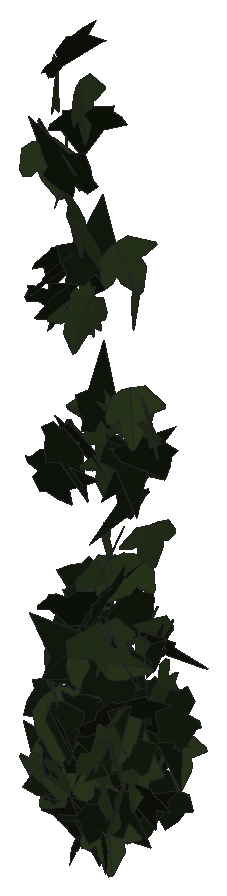
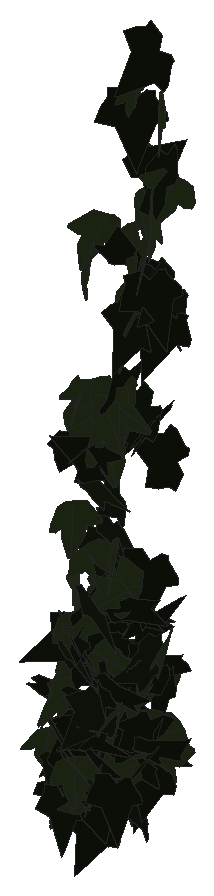
# SketchUp Ruby script. Lengths in inches.
U = 1.inch
M = Sketchup.active_model
def pt(a) = Geom::Point3d.new(a.map { |v| v * U })
def face(e, loops, mat)
  f = e.add_face(loops[0].map { |a| pt(a) })
  loops[1..].each { |l| e.add_face(l.map { |a| pt(a) }).erase! }
  f.material = f.back_material = mat if mat
  f
end
# faces: each face lists its corners as indices into pts; further lists are holes
def faces(e, pts, list, mat = nil) = list.each { |f| face(e, (f[0].is_a?(Array) ? f : [f]).map { |l| l.map { |i| pts[i] } }, mat) }
# xy, xz, yz: faces in a plane at the given z, y or x. An outline is a flat list of corners, or four numbers for a rectangle; further outlines are holes
def ring(l) = l.size == 4 ? [[l[0], l[1]], [l[2], l[1]], [l[2], l[3]], [l[0], l[3]]] : l.each_slice(2).to_a
def flat(e, list, mat, &to3) = list.each { |f| face(e, (f[0].is_a?(Array) ? f : [f]).map { |l| ring(l).map { |u, v| to3.(u, v) } }, mat) }
def xy(e, z, list, mat = nil) = flat(e, list, mat) { |x, y| [x, y, z] }
def xz(e, y, list, mat = nil) = flat(e, list, mat) { |x, z| [x, y, z] }
def yz(e, x, list, mat = nil) = flat(e, list, mat) { |y, z| [x, y, z] }
def lines(e, pts, list) = list.each { |a, b| e.add_line(pt(pts[a]), pt(pts[b])) }
# prism: a flat outline (further loops are holes) pulled along v
def prism(e, loops, v, mat = nil)
  f = face(e, loops, mat); d = Geom::Vector3d.new(v.map { |x| x * U })
  f.pushpull(f.normal.samedirection?(d) ? d.length : -d.length)
end
def box(e, o, s, mat = nil) = prism(e, [[o, [o[0] + s[0], o[1], o[2]], [o[0] + s[0], o[1] + s[1], o[2]], [o[0], o[1] + s[1], o[2]]]], [0, 0, s[2]], mat)
def at(x, y, z, deg = 0) = Geom::Transformation.translation(pt([x, y, z])) * Geom::Transformation.rotation(ORIGIN, Z_AXIS, deg.degrees)
def axes(o, x, y, z) = Geom::Transformation.new([*x, 0, *y, 0, *z, 0, *pt(o).to_a, 1])
def part(name) = M.definitions.add(name)
# library, detail: a bought-in or finely detailed component or shape, given as its bounding box
def library(name, o, s) = part(name).tap { |d| box(d.entities, o, s) }
def detail(e, o, s) = box(e.add_group.entities, o, s)
def put(e, d, t, mat = nil) = e.add_instance(d, t).tap { |i| i.material = mat if mat }
def group(e, t, mat = nil) = e.add_group.tap { |g| g.transformation = t; g.material = mat if mat }.entities
root = M.entities
M.materials.add("efeu1").color = [18, 25, 13]
M.materials.add("efeu2").color = [43, 57, 29]
c1 = part("ivyleaf_9")
p = [[1.54,2.16,1.25],[1.36,2.04,1.19],[-0.21,0.99,0.68],[-0.71,1.11,0.82],[-0.85,0.86,0.67],[-0.8,0.17,0.21],
  [-0.9,-0.01,0.1],[-0.67,-0.16,-0.02],[-0.08,-0.08,-0.05],[-0.03,-0.6,-0.4],[0.65,-0.88,-0.66],[0.83,-0.6,-0.49],
  [1.29,-0.42,-0.43],[1.8125,-0.07,-0.26],[1.21,0.44,0.15]]
faces(c1.entities,p,[[0,1,2,3,4,5,6,7,8,9,10,11,12,13,14]],"efeu1")
c2 = part("ivyleaf_10")
p = [[0,0.5,-0.03],[-0.0625,2.02,-0.43],[-0.19,2.01,-0.46],[-0.54,1.05,-0.29],[-0.52,0.625,-0.18],[-0.83,0.76,-0.28],
  [-1.16,0.64,-0.33],[-1.15,0.33,-0.24],[-0.77,-0.39,0.02],[-0.3,-0.51,0.16],[0.04,-0.48,0.23],[-0.02,2.01,-0.4375],
  [-0.06,2.01,-0.43],[0.04,-0.49,0.23],[0.67,-0.49,0.14],[1.38,0.36,-0.2],[1.375,0.51,-0.24],[0.81,0.65,-0.19],
  [0.62,0.59,-0.15],[0.6,1.09,-0.28],[0.5,1.23,-0.31]]
faces(c2.entities,p,[[0,1,2,3,4,5,6,7,8,9,10],[11,12,0,13,14,15,16,17,18,19,20]],"efeu2")
put(root,c1,axes([595.7,132.61,221.26],[0.61843,0.19992,-0.65752],[0.5583,0.36966,0.6375],[0.40075,-0.82349,0.12654]))
put(root,c1,axes([596.42,132.42,211.24],[0.6186,0.02599,-0.70031],[-0.70079,0.02539,-0.61808],[0.00184,0.93405,0.03629]))
put(root,c2,axes([597.6,132.64,237.72],[-0.15553,0.96808,0.05591],[-0.16512,0.02935,-0.96766],[-0.95553,-0.16265,0.15812]))
put(root,c1,axes([596.97,132.85,233.73],[0.29683,-0.2504,0.90511],[-0.73976,0.52241,0.38713],[-0.57851,-0.7965,-0.03063]))
put(root,c1,axes([596.41,132.97,222.94],[0.35984,-0.79144,-0.21218],[-0.07984,0.19676,-0.86936],[0.81549,0.36849,0.00851]))
put(root,c2,axes([599,132.77,211.11],[-0.33131,0.80604,-0.08092],[0.03205,-0.07431,-0.87147],[-0.80945,-0.33285,-0.00139]))
put(root,c1,axes([598.93,132.13,218.41],[0.07714,0.37838,0.81761],[0.02718,0.81925,-0.3817],[-0.90051,0.05715,0.05852]))
put(root,c2,axes([597.32,133.06,228.49],[-0.38382,-0.85515,0.18299],[0.01116,-0.20461,-0.93279],[0.87444,-0.37275,0.09223]))
put(root,c1,axes([596.29,133.07,212.09],[-0.25767,-0.78685,-0.38038],[0.13269,0.35675,-0.82785],[0.86384,-0.2895,0.0137]))
put(root,c2,axes([598.23,132.98,214.91],[0.74173,-0.52897,-0.04758],[-0.03918,0.027,-0.91103],[0.52966,0.74277,-0.00076]))
put(root,c2,axes([599.05,133.17,211.96],[0.1863,-0.80974,0.20425],[0.07096,-0.19317,-0.83052],[0.83209,0.19776,0.02509]))
put(root,c1,axes([598.87,132.48,217.11],[-0.32407,0.7781,0.31895],[-0.13152,0.29071,-0.84284],[-0.83058,-0.34963,0.00901]))
put(root,c1,axes([597.6,132.69,236.79],[0.3814,0.79106,-0.38325],[-0.16707,-0.34492,-0.8782],[-0.86299,0.41639,0.00064]))
put(root,c2,axes([596.26,132.87,208.13],[-0.27912,0.08871,-0.9003],[-0.86725,0.24188,0.29271],[0.25745,0.91101,0.00995]))
put(root,c1,axes([598.51,132.35,212],[0.37329,0.7726,0.26468],[0.13635,0.22798,-0.85776],[-0.80522,0.39677,-0.02254]))
put(root,c2,axes([596.26,132.61,211.67],[0.35183,0.74282,0.48682],[0.20948,0.43945,-0.82192],[-0.86307,0.40947,-0.00104]))
put(root,c2,axes([598.51,132.9375,208.22],[-0.5257,0.6965,-0.0657],[-0.043,0.04986,0.87262],[0.69827,0.52744,0.00427]))
put(root,c1,axes([598.08,133.62,209.78],[0.54017,-0.75662,-0.18939],[0.11202,-0.15273,0.92966],[-0.77188,-0.55166,0.00238]))
put(root,c2,axes([599.15,133.33,211.57],[0.1387,0.7117,-0.47499],[-0.08904,-0.46658,-0.72509],[-0.85101,0.16481,-0.00155]))
put(root,c2,axes([597.69,132.59,214.03],[0.01969,-0.0615,1.20762],[0.92268,0.78139,0.02475],[-0.78153,0.92096,0.05964]))
put(root,c2,axes([598.45,132.57,211.09],[0.11863,-0.46681,-0.71885],[0.1401,0.7265,-0.44866],[0.8456,-0.05488,0.17518]))
put(root,c1,axes([596.83,133.39,213.43],[-0.37465,-0.80415,-0.06824],[0.00814,-0.079,0.88622],[-0.807,0.37253,0.04062]))
put(root,c2,axes([595.79,133.03,213.2],[-0.29188,0.84168,-0.10173],[0.04981,-0.09038,-0.89068],[-0.84634,-0.29559,-0.01734]))
put(root,c1,axes([596.82,132.83,223.32],[0.8956,-0.04438,-0.25493],[-0.25463,0.01244,-0.8967],[0.04609,0.93109,-0.00017]))
put(root,c1,axes([598.55,133.33,213.6],[-0.153,-0.79125,-0.28943],[0.07252,0.2807,-0.80573],[0.8394,-0.16847,0.01686]))
put(root,c2,axes([598.4,133.08,207.06],[0.72703,0.46011,0.12325],[0.10145,0.07016,-0.86037],[-0.4654,0.73405,0.00498]))
put(root,c1,axes([597.97,133.78,214.14],[-0.02878,-0.25717,-0.90601],[-0.11343,-0.89889,0.25875],[-0.93495,0.11697,-0.0035]))
put(root,c1,axes([596.84,132.77,216.29],[0.4359,0.73963,-0.28028],[-0.20533,-0.20323,-0.85566],[-0.76384,0.47672,0.07007]))
put(root,c1,axes([596.72,132.92,228.87],[-0.6156,0.73662,0.11423],[-0.07071,0.08978,-0.95998],[-0.74207,-0.61964,-0.00329]))
put(root,c2,axes([598.73,133.64,208.15],[-0.08938,0.44318,-0.72072],[-0.02973,-0.72593,-0.44269],[-0.84556,-0.02133,0.09175]))
put(root,c1,axes([598.16,132.89,207.03],[0.25017,-0.00382,-0.87619],[-0.87589,0.02336,-0.25018],[0.02351,0.91091,0.00274]))
put(root,c2,axes([597.22,132.78,232.36],[0.48681,-0.20817,-0.77527],[-0.4737,0.65749,-0.47399],[0.64806,0.63697,0.23589]))
put(root,c1,axes([599.43,133.625,210.85],[-0.77023,-0.30032,0.21904],[-0.19014,-0.11474,-0.8259],[0.31941,-0.79251,0.03657]))
put(root,c1,axes([596.75,132.375,239.17],[0.2871,0.71555,0.64589],[0.2534,0.5942,-0.77092],[-0.93004,0.38278,-0.01066]))
put(root,c1,axes([598.4,132.82,208.1],[-0.02814,-0.26209,-0.82208],[0.07749,0.81842,-0.26357],[0.85936,-0.08238,-0.00315]))
put(root,c2,axes([595.66,133,209.21],[-0.36264,-0.14399,-1.02714],[0.99933,0.24278,-0.38685],[0.27766,-1.06188,0.05083]))
put(root,c1,axes([596.71,133.06,210.77],[-0.31158,-0.00758,0.87739],[0.87694,0.02833,0.31167],[-0.02923,0.93064,-0.00234]))
put(root,c1,axes([595.21,133.82,234.3],[0.719,-0.14985,-0.80959],[0.80152,-0.11846,0.73375],[-0.18832,-1.07627,0.03197]))
put(root,c1,axes([596.44,133.06,207.4],[0.74137,0.41652,-0.33452],[-0.28126,-0.18216,-0.85014],[-0.45419,0.79269,-0.01959]))
put(root,c1,axes([596.17,133.43,208.29],[-0.78324,-0.36423,-0.23745],[-0.21534,-0.10007,0.86379],[-0.37773,0.8123,-0.00006]))
put(root,c1,axes([596.96,133.6,207.79],[-0.47743,-0.28754,-0.72092],[0.62271,0.36331,-0.55729],[0.46329,-0.78464,0.00614]))
put(root,c2,axes([595.77,133.3125,237.53],[0.54417,-0.72711,-0.33694],[0.00531,0.41054,-0.87737],[0.80137,0.49103,0.23461]))
put(root,c2,axes([595.22,133.32,234.15],[0.81744,0.29444,0.36822],[0.26114,0.33087,-0.84429],[-0.39254,0.83326,0.20514]))
put(root,c2,axes([597.2,133.39,228.16],[0.02323,0.09075,0.95466],[-0.95601,0.07709,0.01593],[-0.07522,-0.95183,0.09231]))
put(root,c1,axes([595.96,134,208.32],[0.28637,-0.78905,0.23918],[0.09984,-0.21814,-0.8392],[0.81843,0.3027,0.01869]))
put(root,c2,axes([597.77,133.42,209.63],[-0.73179,-0.35797,-0.32384],[0.27943,0.16543,-0.8143],[0.39361,-0.78295,-0.02399]))
put(root,c1,axes([595.65,132.85,229.2],[0.314,0.66158,0.60187],[0.07416,0.61643,-0.71627],[-0.89131,0.28435,0.15244]))
put(root,c2,axes([598,133.75,214.79],[0.66459,0.05931,0.54121],[0.53947,0.04351,-0.66722],[-0.07347,0.85598,-0.00359]))
put(root,c2,axes([599.29,133.87,209.73],[0.14123,0.77284,-0.3112],[-0.04905,-0.30738,-0.78561],[-0.8317,0.14937,-0.00652]))
put(root,c2,axes([598.8125,133.29,231.12],[0.37179,0.76775,0.46826],[-0.00591,0.50878,-0.82949],[-0.89926,0.31407,0.19905]))
put(root,c2,axes([597.24,133.46,231.21],[-0.71383,0.38656,0.51369],[-0.49305,0.16341,-0.80812],[-0.41256,-0.86414,0.07698]))
put(root,c2,axes([597.6,134.21,223.11],[-0.44993,-0.59437,-0.53274],[-0.32336,-0.42339,0.74546],[-0.72975,0.55407,-0.00186]))
put(root,c1,axes([597.48,133.47,229.95],[-0.89478,0.0678,0.30911],[0.30852,-0.0194,0.89734],[0.07042,0.94647,-0.00375]))
put(root,c1,axes([599.12,133.3,212.25],[0.56653,0.66139,0.01987],[0.01313,0.01492,-0.87085],[-0.66156,0.56668,-0.00027]))
put(root,c1,axes([598.18,133.56,211.09],[0.75048,-0.22593,-0.36094],[-0.32857,0.158,-0.78206],[0.27086,0.81764,0.05139]))
put(root,c1,axes([595.87,133.8125,212.73],[0.76247,-0.40376,0.16957],[0.15157,-0.07612,-0.86277],[0.41086,0.77738,0.00359]))
put(root,c2,axes([598.77,134.36,229.38],[0.11871,-0.36931,0.83747],[0.62301,-0.58605,-0.34675],[0.67052,0.60991,0.17392]))
put(root,c1,axes([596.09,133.65,209.84],[-0.00033,-0.53595,-0.70786],[0.12859,0.70037,-0.53033],[0.87851,-0.10271,0.07736]))
put(root,c2,axes([596.89,133.5,209.17],[0.35522,0.24862,1.05811],[0.90515,0.54863,-0.43278],[-0.60176,0.972,-0.02637]))
put(root,c1,axes([599.26,133.57,208.82],[0.7364,0.27505,-0.37064],[-0.35882,-0.09781,-0.78549],[-0.29031,0.81859,0.03069]))
put(root,c1,axes([597.66,133.59,223.84],[-0.26343,-0.52387,0.74316],[0.32738,0.66718,0.58636],[-0.84826,0.42018,-0.00449]))
put(root,c1,axes([597.83,134.33,214.42],[0.36254,-0.69829,0.3383],[0.20501,-0.27393,-0.78513],[0.74835,0.41333,0.05119]))
put(root,c2,axes([598.03,134.21,212.4],[0.40834,0.21576,-0.7096],[-0.66859,-0.24356,-0.45879],[-0.32105,0.78164,0.05292]))
put(root,c2,axes([597.9,134.14,222],[-0.38747,-0.83117,0.14025],[-0.06307,-0.12534,-0.91704],[0.84056,-0.39254,-0.00415]))
put(root,c1,axes([596.92,133.41,208.85],[0.14702,0.08202,0.89432],[0.69051,0.5691,-0.16571],[-0.57421,0.70537,0.0297]))
put(root,c1,axes([595.27,133.61,228.25],[0.6862,0.58326,-0.16906],[-0.15363,-0.08006,-0.89979],[-0.58751,0.70217,0.03784]))
put(root,c2,axes([596.14,133.92,231.06],[-0.59048,0.7259,0.0234],[-0.05322,-0.01317,-0.93442],[-0.72432,-0.59079,0.04958]))
put(root,c2,axes([597.47,134.06,223.67],[-0.15115,0.0275,0.90868],[-0.9007,-0.12943,-0.14591],[0.12327,-0.91203,0.0481]))
put(root,c1,axes([596.71,133.46,205.66],[0.06983,0.26703,0.89686],[-0.08368,0.89753,-0.26072],[-0.93202,-0.06057,0.09061]))
put(root,c1,axes([598.32,133.61,217],[0.01574,0.82906,0.25265],[-0.09851,0.25277,-0.8233],[-0.86109,-0.01376,0.0988]))
put(root,c1,axes([598.16,134.59,222.1],[0.11028,-0.88447,0.1392],[0.1333,-0.12247,-0.88377],[0.88537,0.1286,0.11573]))
put(root,c1,axes([597.93,134.2,213.375],[-0.20612,-0.40809,-0.74835],[0.49636,0.56845,-0.4467],[0.69296,-0.52857,0.09737]))
put(root,c1,axes([595.69,134.12,229.91],[0.02349,0.84962,-0.38675],[-0.04405,-0.38543,-0.8494],[-0.93246,0.03961,0.03038]))
put(root,c1,axes([596.88,134.77,215.17],[-0.72378,-0.44948,0.19428],[-0.16498,-0.10259,-0.85199],[0.46104,-0.74234,0.00011]))
put(root,c2,axes([596.86,133.67,207.62],[0.06053,-0.10299,0.88676],[0.07315,0.88638,0.09795],[-0.88972,0.06587,0.06838]))
put(root,c1,axes([598.49,134.73,220.42],[-0.79209,0.16266,-0.36138],[0.26724,-0.37717,-0.7555],[-0.29264,-0.78469,0.28823]))
put(root,c1,axes([597.88,133.8,209.58],[0.57685,0.08993,0.64163],[0.5087,0.46919,-0.52309],[-0.40126,0.72409,0.25926]))
put(root,c2,axes([598.46,134.36,224.43],[0.47758,0.77237,0.01431],[0.00689,0.01256,-0.90809],[-0.77247,0.47763,0.00075]))
put(root,c1,axes([598.92,134.81,222.32],[-0.02441,0.36675,-0.81999],[-0.0175,-0.82033,-0.36639],[-0.8981,0.00602,0.02942]))
put(root,c2,axes([599.46,134.06,214.95],[-0.06185,0.3997,0.77683],[-0.65188,0.49735,-0.3078],[-0.58161,-0.59995,0.26238]))
put(root,c2,axes([597.36,134.63,223.43],[0.07374,0.86154,-0.25574],[-0.30901,-0.21665,-0.81894],[-0.8439,0.15461,0.27753]))
put(root,c2,axes([598.8125,134.74,222.73],[-0.5723,0.05512,-0.68237],[-0.68206,-0.12231,0.56217],[-0.05881,0.88216,0.12058]))
put(root,c2,axes([598.18,134.84,217.17],[0.51958,0.48892,-0.49857],[-0.45945,-0.22863,-0.703],[-0.52585,0.68284,0.12161]))
put(root,c1,axes([596.21,135.21,215.58],[-0.64774,-0.49461,0.22946],[-0.17238,-0.15228,-0.81484],[0.51728,-0.6701,0.0158]))
put(root,c2,axes([598.9,134.74,224.04],[-0.53949,0.69521,-0.22127],[0.13311,-0.17679,-0.87997],[-0.71733,-0.55566,0.00313]))
put(root,c2,axes([596.45,134.31,227.84],[-0.42803,0.64043,0.51265],[-0.27686,0.43153,-0.77025],[-0.7722,-0.50971,-0.00799]))
put(root,c2,axes([596.66,134.1875,215.98],[-0.00749,-0.14571,0.87284],[0.25266,0.83619,0.14176],[-0.84809,0.2504,0.03453]))
put(root,c2,axes([595.48,134.21,233.34],[0.21728,-0.55686,-0.98749],[-0.33635,0.92853,-0.59762],[1.08264,0.40024,0.01252]))
put(root,c1,axes([597.76,134.41,221.3],[0.01111,-0.03866,0.90995],[0.8255,0.38487,0.00627],[-0.38476,0.82462,0.03973]))
put(root,c1,axes([597.21,135.3,212.07],[-0.43179,0.21164,-0.70348],[0.62859,-0.31587,-0.48086],[-0.3802,-0.7626,0.00393]))
put(root,c2,axes([598.91,134.98,218.83],[-0.42344,-0.76141,-0.08895],[0.05095,0.07344,-0.87119],[0.76489,-0.4264,0.00879]))
put(root,c2,axes([596.97,134.8,217.78],[-0.49924,0.61751,0.39235],[-0.29723,0.26284,-0.79188],[-0.66852,-0.57801,0.05907]))
put(root,c1,axes([596.15,134.48,228.26],[0.19579,0.81669,0.3692],[0.06201,0.36466,-0.83952],[-0.89412,0.20413,0.02262]))
put(root,c1,axes([598.84,135.47,214],[-0.71857,0.277,-0.35839],[0.32828,-0.1446,-0.76996],[-0.3121,-0.78986,0.01527]))
put(root,c1,axes([598.06,135.27,214.72],[-0.29337,-0.7251,0.4018],[0.14857,0.37333,0.7822],[-0.81557,0.32884,-0.00204]))
put(root,c1,axes([598.17,135.67,206.83],[-0.76563,-0.13707,0.21901],[-0.21385,-0.04815,-0.77774],[0.14498,-0.79488,0.00934]))
put(root,c1,axes([599,135.7,210.39],[0.2834,-0.79481,0.06296],[0.0355,-0.05417,-0.84369],[0.79651,0.28521,0.0152]))
put(root,c1,axes([599.85,135.77,211.13],[-0.79496,-0.09923,0.27915],[-0.26265,-0.13375,-0.79552],[0.13706,-0.83186,0.09461]))
put(root,c1,axes([598.65,135.9,211.08],[-0.73441,-0.36202,0.18741],[-0.15941,-0.10037,-0.81857],[0.3752,-0.75127,0.01905]))
put(root,c2,axes([596.36,135.43,210.86],[-0.1143,0.81485,-0.0705],[0.00165,-0.07096,-0.82279],[-0.8179,-0.11402,0.00819]))
put(root,c1,axes([598.5,134.95,207.18],[0.38837,0.66938,0.24934],[0.12811,0.21394,-0.77388],[-0.70273,0.40894,-0.00328]))
put(root,c2,axes([596.34,135.24,216.11],[0.36835,0.27576,0.71285],[0.50958,0.50119,-0.45719],[-0.56967,0.62662,0.05197]))
put(root,c2,axes([598.35,135.61,214.34],[-0.38173,-0.77141,-0.05585],[0.05423,0.03544,-0.86007],[0.77153,-0.38417,0.03282]))
put(root,c1,axes([597.24,135.22,208.55],[0.43575,-0.12541,-0.70487],[-0.63205,0.3202,-0.4477],[0.33628,0.76433,0.0719]))
put(root,c1,axes([596.46,135.55,211.88],[-0.19826,0.34186,0.72642],[-0.66367,0.35125,-0.34644],[-0.45177,-0.66605,0.19014]))
put(root,c1,axes([597.6875,135.42,208.38],[-0.24425,0.32299,0.75742],[-0.53751,0.53596,-0.40188],[-0.62378,-0.5883,0.04972]))
put(root,c1,axes([598.12,135.26,209.22],[0.50844,0.55737,0.33393],[0.24333,0.22982,-0.75409],[-0.60246,0.56321,-0.02275]))
put(root,c1,axes([599.05,135.96,209.7],[-0.70874,0.36783,-0.19995],[0.18341,-0.0806,-0.7984],[-0.37635,-0.73198,-0.01257]))
put(root,c1,axes([597.58,135.83,207.15],[-0.02801,0.68229,-0.44682],[-0.1118,-0.44607,-0.67415],[-0.80788,0.03808,0.10878]))
put(root,c1,axes([598.69,135.86,213.6],[-0.66628,0.5246,-0.03584],[0.01847,-0.03447,-0.84788],[-0.5255,-0.66636,0.01564]))
put(root,c2,axes([598.95,135.45,212.29],[0.13841,-0.51456,-0.6732],[0.04014,0.68534,-0.51558],[0.84638,0.05164,0.13454]))
put(root,c1,axes([598.86,136.35,207.39],[-0.12178,-0.20705,-0.77913],[-0.3657,-0.68805,0.24],[-0.71846,0.38531,0.0099]))
put(root,c1,axes([598.23,135.61,213.75],[0.79865,0.01676,0.27768],[0.27256,0.12166,-0.79129],[-0.05562,0.83674,0.10949]))
put(root,c1,axes([597.33,136.51,209.78],[-0.39703,-0.71602,0.01437],[0.1366,-0.09184,-0.80214],[0.70302,-0.38652,0.16397]))
put(root,c1,axes([597.37,135.86,215.99],[-0.52036,0.67298,0.02417],[-0.01239,0.02097,-0.85068],[-0.6733,-0.5205,-0.00303]))
put(root,c1,axes([598.22,135.79,208.28],[-0.32894,0.58478,0.46485],[-0.38354,0.30366,-0.65341],[-0.64105,-0.48175,0.15241]))
put(root,c1,axes([597.36,136.49,209.93],[-0.73623,-0.13506,0.33056],[-0.31392,-0.11623,-0.74666],[0.1702,-0.79862,0.05276]))
put(root,c1,axes([595.93,135.97,208],[0.11514,0.79053,-0.16015],[-0.025,-0.1582,-0.79887],[-0.8062,0.1178,0.0019]))
put(root,c1,axes([596.875,135.81,206.02],[0.44763,0.67684,0.04547],[0.02237,0.03971,-0.81147],[-0.678,0.44818,0.00324]))
put(root,c1,axes([598.64,136.21,208.38],[-0.39556,0.69438,-0.16098],[-0.09195,-0.23228,-0.77598],[-0.70684,-0.35837,0.19103]))
put(root,c2,axes([599.17,136.23,209.36],[0.24813,0.78233,-0.00714],[-0.02277,-0.00027,-0.82046],[-0.78204,0.24823,0.02162]))
put(root,c1,axes([596.75,135.89,211.19],[0.6107,0.50027,0.21872],[0.02301,0.30429,-0.76022],[-0.5455,0.57289,0.21279]))
put(root,c2,axes([598.55,135.88,211.24],[-0.00929,0.37561,0.74869],[-0.10646,0.74214,-0.37364],[-0.83084,-0.0993,0.03951]))
put(root,c2,axes([597.6,136.57,208.51],[-0.61495,-0.52078,0.05718],[-0.01695,-0.06834,-0.80479],[0.52364,-0.61381,0.04109]))
put(root,c2,axes([597.57,136.78,206.82],[0.39366,0.57876,-0.39505],[-0.2167,-0.33036,-0.69993],[-0.66639,0.44933,-0.00577]))
put(root,c1,axes([597.9,136.86,207.13],[-0.01456,0.79464,0.0476],[0.00454,0.04769,-0.79475],[-0.79605,-0.01426,-0.0054]))
